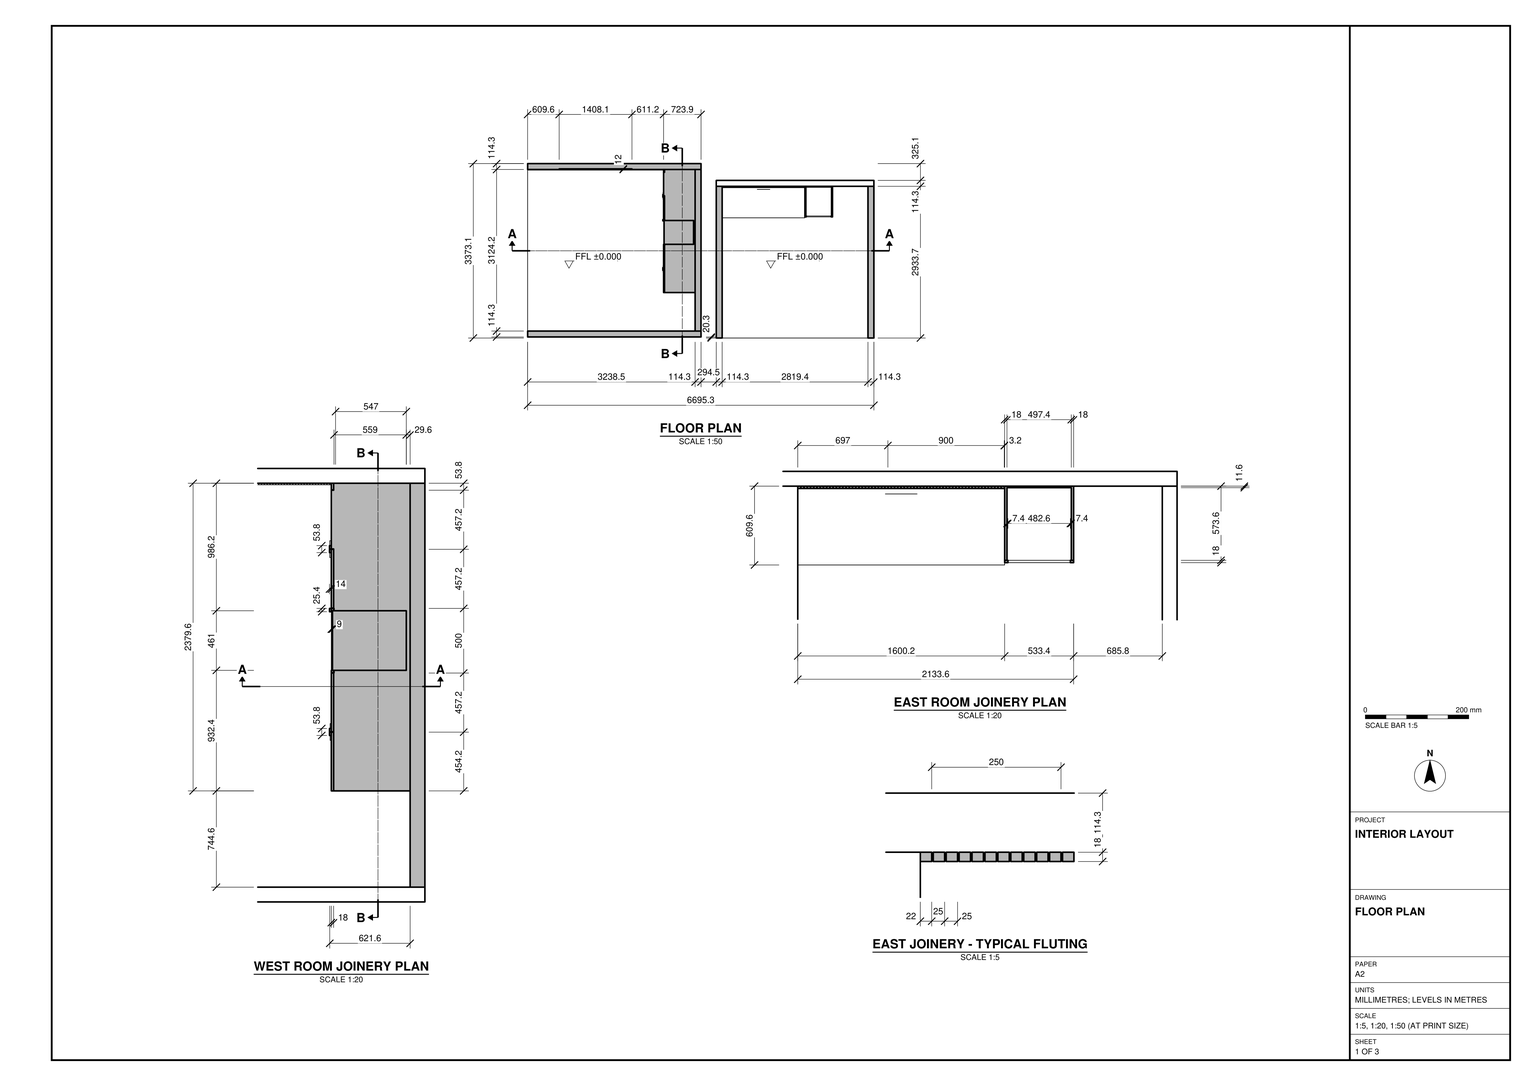
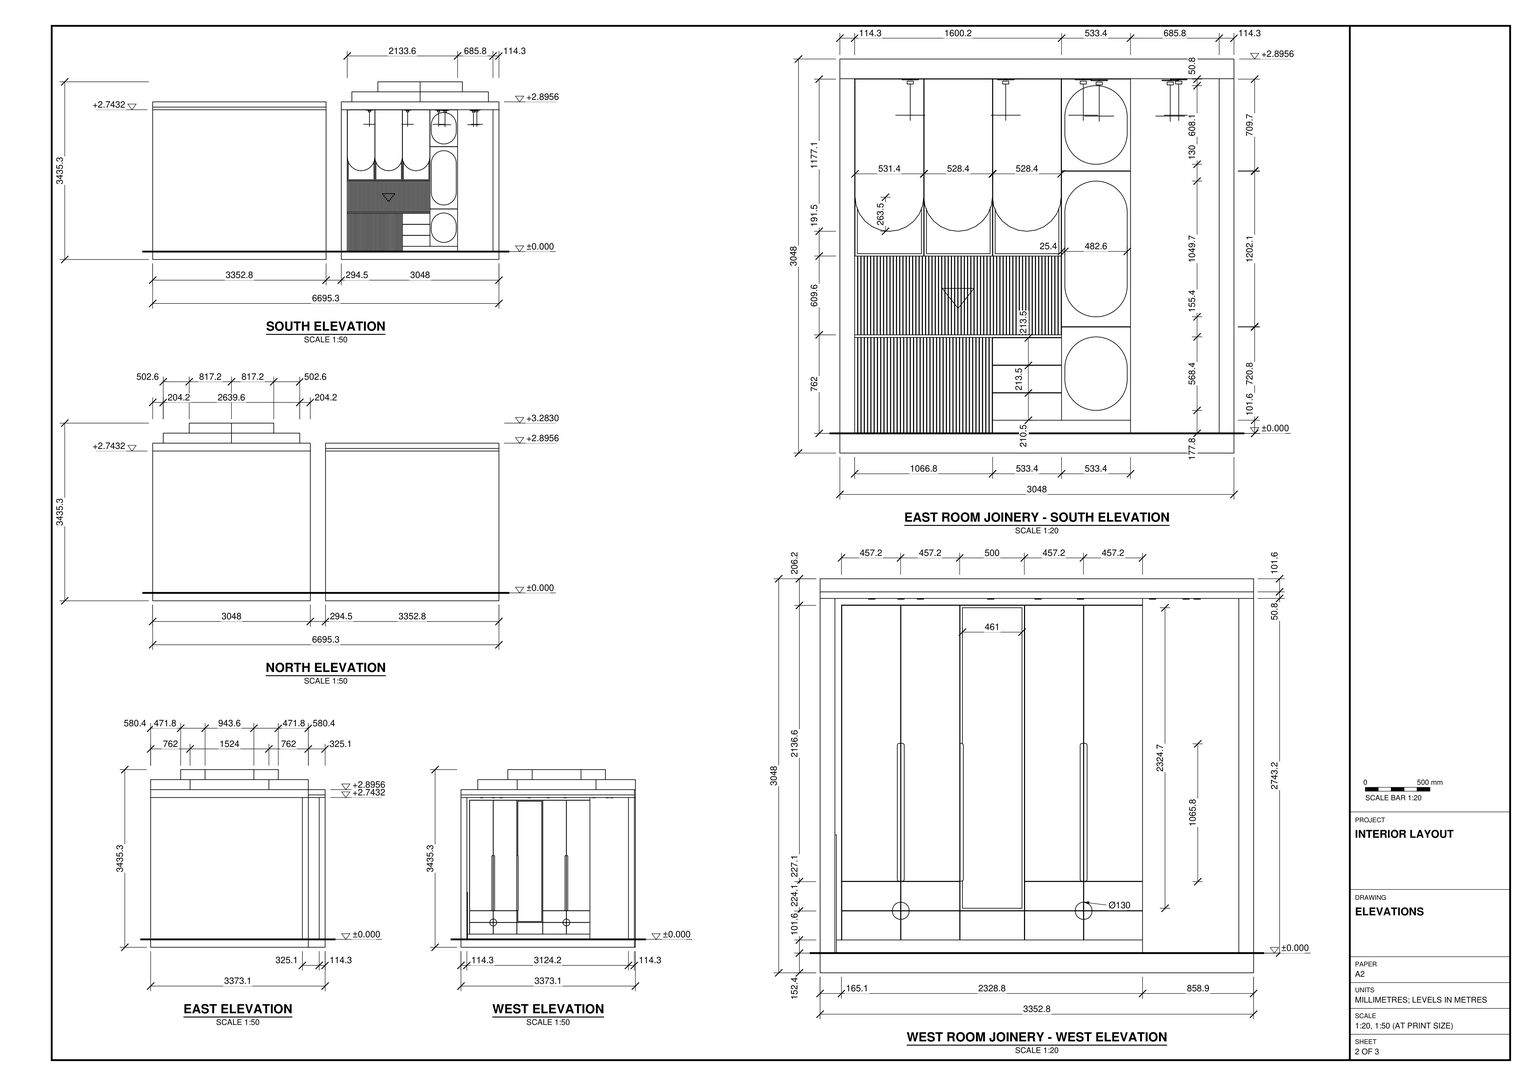
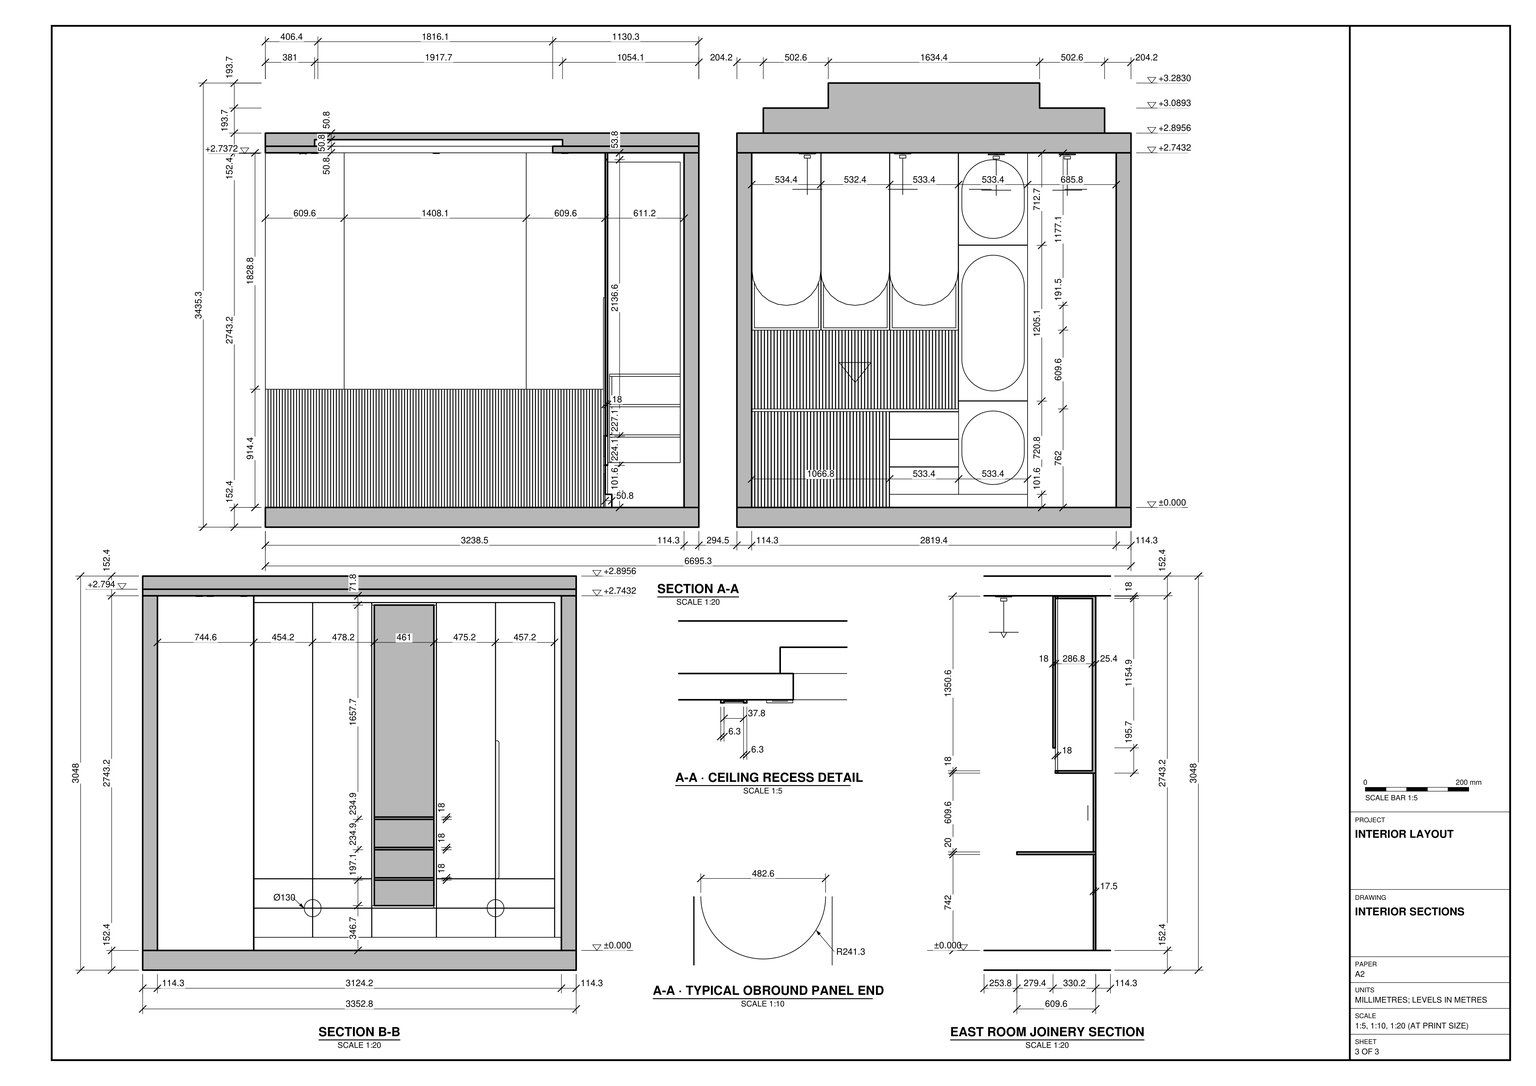
Build the west and east room bays in SketchUp from task_files/diagram_01.pdf. Work in millimetres. The overall model is 6695.3 mm along X, 3373.1 mm along Y and 3435.3 mm high. Both bays have the same finished floor level, ±0.000 (0 mm). Align their south edges, leave the 294.5 mm gap between the shells and set the north edge of the east bay back as drawn. Model the floor slabs, 114.3 mm walls and overhead construction, keeping the west bay open to the west and the east bay open to the south. Follow the sections for the west ceiling recess and the stepped top over the east bay.

Fit the tall storage unit against the east wall of the west bay. Model the paired tall fronts, long pulls, divided lower fronts and framed central bay with its internal shelves. Include the fluted lower wall lining visible in section A-A. Against the north wall of the east bay, build the joinery shown in the south elevation: rounded lower ends on the upper panels, a fluted middle band, a projecting work surface, divided fronts below and a narrow side column with obround panels. Use the enlarged details for the fluting and curved ends. Decor and loose items, including light fixtures, may be any suitable library components placed as shown.

Keep the shell elements and each furniture or joinery piece in separate groups or components, and make repeated parts components. Save one SketchUp model as output_files/two_interior_bays_with_fitted_wall_joinery.skp.

# SketchUp Ruby script. Lengths in millimetres.
U = 1.mm
M = Sketchup.active_model
def pt(a) = Geom::Point3d.new(a.map { |v| v * U })
def face(e, loops, mat)
  f = e.add_face(loops[0].map { |a| pt(a) })
  loops[1..].each { |l| e.add_face(l.map { |a| pt(a) }).erase! }
  f.material = f.back_material = mat if mat
  f
end
# faces: each face lists its corners as indices into pts; further lists are holes
def faces(e, pts, list, mat = nil) = list.each { |f| face(e, (f[0].is_a?(Array) ? f : [f]).map { |l| l.map { |i| pts[i] } }, mat) }
# xy, xz, yz: faces in a plane at the given z, y or x. An outline is a flat list of corners, or four numbers for a rectangle; further outlines are holes
def ring(l) = l.size == 4 ? [[l[0], l[1]], [l[2], l[1]], [l[2], l[3]], [l[0], l[3]]] : l.each_slice(2).to_a
def flat(e, list, mat, &to3) = list.each { |f| face(e, (f[0].is_a?(Array) ? f : [f]).map { |l| ring(l).map { |u, v| to3.(u, v) } }, mat) }
def xy(e, z, list, mat = nil) = flat(e, list, mat) { |x, y| [x, y, z] }
def xz(e, y, list, mat = nil) = flat(e, list, mat) { |x, z| [x, y, z] }
def yz(e, x, list, mat = nil) = flat(e, list, mat) { |y, z| [x, y, z] }
def lines(e, pts, list) = list.each { |a, b| e.add_line(pt(pts[a]), pt(pts[b])) }
# prism: a flat outline (further loops are holes) pulled along v
def prism(e, loops, v, mat = nil)
  f = face(e, loops, mat); d = Geom::Vector3d.new(v.map { |x| x * U })
  f.pushpull(f.normal.samedirection?(d) ? d.length : -d.length)
end
def box(e, o, s, mat = nil) = prism(e, [[o, [o[0] + s[0], o[1], o[2]], [o[0] + s[0], o[1] + s[1], o[2]], [o[0], o[1] + s[1], o[2]]]], [0, 0, s[2]], mat)
def at(x, y, z, deg = 0) = Geom::Transformation.translation(pt([x, y, z])) * Geom::Transformation.rotation(ORIGIN, Z_AXIS, deg.degrees)
def axes(o, x, y, z) = Geom::Transformation.new([*x, 0, *y, 0, *z, 0, *pt(o).to_a, 1])
def part(name) = M.definitions.add(name)
# library, detail: a bought-in or finely detailed component or shape, given as its bounding box
def library(name, o, s) = part(name).tap { |d| box(d.entities, o, s) }
def detail(e, o, s) = box(e.add_group.entities, o, s)
def put(e, d, t, mat = nil) = e.add_instance(d, t).tap { |i| i.material = mat if mat }
def group(e, t, mat = nil) = e.add_group.tap { |g| g.transformation = t; g.material = mat if mat }.entities
root = M.entities
M.materials.add("Olon-Denim-Chic-VT14-1K").color = [84, 100, 105]
M.materials.add("Olon-Fresh-Linen-VT10-1K").color = [226, 220, 209]
M.materials.add("Pionite-a-Panolam-Brand-Canyon-Shadow-SO200-4K").color = [135, 86, 67]
M.materials.add("Uniboard-L17-Ambrette-4K").color = [104, 52, 49]
M.materials.add("Uniboard-L19-Putty-4K").color = [187, 181, 160]
M.materials.add("[Color M00]").color = [255, 255, 255]
M.materials.add("[Color M09]1").color = [0, 0, 0]
M.materials.add("[Translucent Glass Gray]").color = [128, 128, 128]
c1 = part("Group280\#1")
p = [[0,0,0],[0,0,-404.7],[-1.4,0,-404.7],[9,-1301.3,0],[-9,-1301.3,0],[9,1301.3,0],
  [9,0,0],[-9,1301.3,0],[1.4,0,-404.7],[-9,0,0],[0,0,-655.2]]
lines(c1.entities,p,[[0,1],[1,2],[3,4],[5,6],[7,5],[1,8],[9,0],[0,6],[8,10],[4,9],[6,3],[2,10],
  [9,7]])
c2 = part("Rectangle Light\#1")
put(c2.entities,c1,at(0,0,0))
c3 = part("Group282\#1")
p = [[0,0,0],[0,0,-404.7],[-1.4,0,-404.7],[9,-1301.3,0],[-9,-1301.3,0],[9,1301.3,0],
  [9,0,0],[-9,1301.3,0],[1.4,0,-404.7],[-9,0,0],[0,0,-655.2]]
lines(c3.entities,p,[[0,1],[1,2],[3,4],[5,6],[7,5],[1,8],[9,0],[0,6],[8,10],[4,9],[6,3],[2,10],
  [9,7]])
c4 = part("Rectangle Light\#2")
put(c4.entities,c3,at(0,0,0))
c5 = part("Group292\#1")
p = [[0,0,0],[0,0,-167.5],[-81.9,0,-167.5],[533.4,-9,0],[-533.4,-9,0],[533.4,9,0],
  [533.4,0,0],[-533.4,9,0],[81.9,0,-167.5],[-533.4,0,0],[0,0,-271.2]]
lines(c5.entities,p,[[0,1],[1,2],[3,4],[5,6],[7,5],[1,8],[9,0],[0,6],[8,10],[4,9],[6,3],[2,10],
  [9,7]])
c6 = part("Rectangle Light\#3")
put(c6.entities,c5,at(0,0,0))
c7 = library("Group10\#1",[-1313.7,-457.2,0],[2627.4,914.4,12])
c8 = library("Group\#3",[-12,435,0],[621.6,2379.6,2743.2])
c9 = part("Group\#6")
prism(c9.entities,[[[0,248.3,178.4],[0,254.5,178.9],[0,259.6,180.5],[0,263.5,183.1],[0,266.3,186.7],[0,268,191.4],[0,268.6,197.1],[0,461,197.1],[0,461,0],[0,0,0],[0,0,197.1],[0,192.4,197.1],[0,193,191.4],[0,194.7,186.7],[0,197.5,183.1],[0,201.4,180.5],[0,206.5,178.9],[0,212.7,178.4]]],[18,0,0])
c10 = part("Group\#7")
prism(c10.entities,[[[20,25.4,1066.8],[20,17.4,1066.8],[20,12.1,1066.3],[20,7.7,1064.9],[20,4.3,1062.5],[20,1.9,1059.1],[20,0.5,1054.7],[20,0,1049.4],[20,0,17.4],[20,0.5,12.1],[20,1.9,7.7],[20,4.3,4.3],[20,7.7,1.9],[20,12.1,0.5],[20,17.4,0],[20,25.4,0]]],[-14,0,0])
c11 = part("Group\#17")
xy(c11.entities,314.6,[[[110.7,87.8,104.3,89.2,98.4,92.3,93.5,96.8,90,102.4,88,108.7,87.8,115.4,89.2,121.8,92.3,127.7,96.8,132.6,102.4,136.1,108.7,138.1,115.4,138.3,121.8,136.9,127.7,133.8,132.6,129.3,136.1,123.7,138.1,117.3,138.3,110.7,136.9,104.3,133.8,98.4,129.3,93.5,123.7,90,117.3,88],[111.3,94.1,116.3,94.3,121,95.7,125.2,98.4,128.6,102.1,130.9,106.5,132,111.3,131.8,116.3,130.3,121,127.7,125.2,124,128.6,119.6,130.9,114.8,132,109.8,131.8,105.1,130.3,100.9,127.7,97.5,124,95.2,119.6,94.1,114.8,94.3,109.8,95.7,105.1,98.4,100.9,102.1,97.5,106.5,95.2]]])
xy(c11.entities,320.6,[[110.7,87.8,117.3,88,123.7,90,129.3,93.5,133.8,98.4,136.9,104.3,138.3,110.7,138.1,117.3,136.1,123.7,132.6,129.3,127.7,133.8,121.8,136.9,115.4,138.3,108.7,138.1,102.4,136.1,96.8,132.6,92.3,127.7,89.2,121.8,87.8,115.4,88,108.7,90,102.4,93.5,96.8,98.4,92.3,104.3,89.2]])
p = [[110.7,87.8,320.6],[104.3,89.2,320.6],[104.3,89.2,314.6],[110.7,87.8,314.6],[117.3,88,320.6],[117.3,88,314.6],
  [123.7,90,320.6],[123.7,90,314.6],[98.4,92.3,320.6],[98.4,92.3,314.6],[129.3,93.5,320.6],[129.3,93.5,314.6],
  [93.5,96.8,320.6],[93.5,96.8,314.6],[133.8,98.4,320.6],[133.8,98.4,314.6],[111.3,94.1,314.6],[106.5,95.2,314.6],
  [106.5,95.2,317.8],[111.3,94.1,317.8],[116.3,94.3,314.6],[116.3,94.3,317.8],[121,95.7,314.6],[121,95.7,317.8],
  [102.1,97.5,314.6],[102.1,97.5,317.8],[125.2,98.4,314.6],[125.2,98.4,317.8],[90,102.4,320.6],[90,102.4,314.6],
  [98.4,100.9,314.6],[98.4,100.9,317.8],[128.6,102.1,314.6],[128.6,102.1,317.8],[136.9,104.3,320.6],[136.9,104.3,314.6],
  [95.7,105.1,314.6],[95.7,105.1,317.8],[130.9,106.5,314.6],[130.9,106.5,317.8],[88,108.7,320.6],[88,108.7,314.6],
  [138.3,110.7,320.6],[138.3,110.7,314.6],[94.3,109.8,314.6],[94.3,109.8,317.8],[132,111.3,314.6],[132,111.3,317.8],
  [87.8,115.4,320.6],[87.8,115.4,314.6],[94.1,114.8,314.6],[94.1,114.8,317.8],[138.1,117.3,320.6],[138.1,117.3,314.6],
  [131.8,116.3,314.6],[131.8,116.3,317.8],[95.2,119.6,314.6],[95.2,119.6,317.8],[89.2,121.8,320.6],[89.2,121.8,314.6],
  [130.3,121,314.6],[130.3,121,317.8],[136.1,123.7,320.6],[136.1,123.7,314.6],[97.5,124,314.6],[97.5,124,317.8],
  [127.7,125.2,314.6],[127.7,125.2,317.8],[92.3,127.7,320.6],[92.3,127.7,314.6],[132.6,129.3,320.6],[132.6,129.3,314.6],
  [100.9,127.7,314.6],[100.9,127.7,317.8],[124,128.6,314.6],[124,128.6,317.8],[96.8,132.6,320.6],[96.8,132.6,314.6],
  [105.1,130.3,314.6],[105.1,130.3,317.8],[119.6,130.9,314.6],[119.6,130.9,317.8],[127.7,133.8,320.6],[127.7,133.8,314.6],
  [109.8,131.8,314.6],[109.8,131.8,317.8],[114.8,132,314.6],[114.8,132,317.8],[102.4,136.1,320.6],[102.4,136.1,314.6],
  [121.8,136.9,320.6],[121.8,136.9,314.6],[108.7,138.1,320.6],[108.7,138.1,314.6],[115.4,138.3,320.6],[115.4,138.3,314.6]]
faces(c11.entities,p,[[0,1,2,3],[4,0,3,5],[6,4,5,7],[1,8,9,2],[10,6,7,11],[8,12,13,9],[14,10,11,15],[16,17,18,19],
  [20,16,19,21],[22,20,21,23],[17,24,25,18],[26,22,23,27],[12,28,29,13],[24,30,31,25],[32,26,27,33],[34,14,15,35],
  [30,36,37,31],[38,32,33,39],[28,40,41,29],[42,34,35,43],[36,44,45,37],[46,38,39,47],[40,48,49,41],[44,50,51,45],
  [52,42,43,53],[54,46,47,55],[50,56,57,51],[48,58,59,49],[60,54,55,61],[62,52,53,63],[56,64,65,57],[66,60,61,67],
  [58,68,69,59],[70,62,63,71],[64,72,73,65],[74,66,67,75],[68,76,77,69],[72,78,79,73],[80,74,75,81],[82,70,71,83],
  [78,84,85,79],[86,80,81,87],[84,86,87,85],[76,88,89,77],[90,82,83,91],[88,92,93,89],[94,90,91,95],[92,94,95,93]])
g1 = group(c11.entities,at(94.1,94.1,317.8))
xy(g1,0,[[17.2,0,12.4,1.1,8,3.4,4.3,6.8,1.7,11,0.2,15.7,0,20.7,1.1,25.6,3.4,30,6.8,33.6,11,36.3,15.7,37.8,20.7,37.9,25.6,36.8,30,34.5,33.6,31.2,36.3,27,37.8,22.2,37.9,17.2,36.8,12.4,34.5,8,31.2,4.3,27,1.7,22.2,0.2]])
c12 = library("Group161\#1",[-800.1,-304.8,0],[1600.2,609.6,18])
c13 = library("Group227\#2",[-533.4,-371,0],[1066.8,742,17.5])
c14 = part("Group278\#1")
p = [[0,0,0],[0,0,-249.9],[-122.9,0,-249.9],[800.1,-9,0],[-800.1,-9,0],[800.1,9,0],
  [800.1,0,0],[-800.1,9,0],[122.9,0,-249.9],[-800.1,0,0],[0,0,-404.6]]
lines(c14.entities,p,[[0,1],[1,2],[3,4],[5,6],[7,5],[1,8],[9,0],[0,6],[8,10],[4,9],[6,3],[2,10],
  [9,7]])
c15 = part("Rectangle Light")
put(c15.entities,c14,at(0,0,0))
c16 = library("Group\#28",[0,0,0],[533.4,18,709.7])
c17 = library("Group\#29",[0,0,0],[533.4,18,1202.1])
c18 = library("Group\#30",[0,0,0],[533.4,18,720.8])
c19 = library("Group\#31",[0,0,0],[226.1,226.1,320.6])
xy(root,3048,[[5171.3,0,3851.4,762,3851.4,2286,5171.3,3048,6491.1,2286,6491.1,762]])
xy(root,3241.7,[[[5171.3,0,6491.1,762,6491.1,2286,5171.3,3048,3851.4,2286,3851.4,762],[5171.3,580.4,4354.1,1052.2,4354.1,1995.8,5171.3,2467.6,5988.4,1995.8,5988.4,1052.2]]])
xy(root,3435.4,[[5171.3,580.4,5988.4,1052.2,5988.4,1995.8,5171.3,2467.6,4354.1,1995.8,4354.1,1052.2]])
yz(root,2637.9,[[1811.6,499.1,2272.6,2823.8]],"[Translucent Glass Gray]")
yz(root,3851.4,[[762,3048,2286,3241.7]])
yz(root,4354.1,[[1052.2,3241.7,1995.8,3435.4]])
yz(root,5988.4,[[1052.2,3241.7,1995.8,3435.4]])
yz(root,6491.1,[[762,3048,2286,3241.7]])
p = [[3851.4,762,3048],[5171.3,0,3048],[5171.3,0,3241.7],[3851.4,762,3241.7],[6491.1,762,3048],[6491.1,762,3241.7],
  [5171.3,3048,3048],[3851.4,2286,3048],[3851.4,2286,3241.7],[5171.3,3048,3241.7],[6491.1,2286,3048],[6491.1,2286,3241.7],
  [4354.1,1052.2,3241.7],[5171.3,580.4,3241.7],[5171.3,580.4,3435.4],[4354.1,1052.2,3435.4],[5988.4,1052.2,3241.7],[5988.4,1052.2,3435.4],
  [5171.3,2467.6,3241.7],[4354.1,1995.8,3241.7],[4354.1,1995.8,3435.4],[5171.3,2467.6,3435.4],[5988.4,1995.8,3241.7],[5988.4,1995.8,3435.4]]
faces(root,p,[[0,1,2,3],[1,4,5,2],[6,7,8,9],[10,6,9,11],[12,13,14,15],[13,16,17,14],[18,19,20,21],[22,18,21,23]])
put(root,c2,axes([5380,2632.1,1573.3],[0,-1,0],[0,0,1],[-1,0,0]))
put(root,c4,axes([5876.9,2632.1,1573.3],[0,-1,0],[0,0,1],[1,0,0]))
put(root,c6,axes([4295,2858.6,894.1],[1,0,0],[0,-1,0],[0,0,1]))
g2 = group(root,at(0,20.3,0))
box(g2,[0,0,0],[3352.8,3352.8,152.4])
g3 = group(root,at(3238.5,134.6,152.4))
box(g3,[0,0,0],[114.3,3124.2,2743.2])
g4 = group(root,at(0,3258.8,152.4),"Uniboard-L19-Putty-4K")
xy(g4,0,[[0,0,3352.8,114.3]])
xy(g4,2743.2,[[0,0,609.6,0,609.6,12,2017.7,12,2017.7,0,3352.8,0,3352.8,114.3,0,114.3]],"[Color M00]")
xz(g4,0,[[2627.3,0,3352.8,2743.2],[0,914.4,609.6,2743.2],[2017.7,914.4,2627.3,2743.2]])
xz(g4,12,[[609.6,914.4,2017.7,2743.2]])
xz(g4,114.3,[[0,0,3352.8,2743.2]],"[Color M00]")
yz(g4,0,[[0,0,114.3,2743.2]],"[Color M00]")
yz(g4,3352.8,[[0,0,114.3,2743.2]],"[Color M00]")
put(g4,c7,axes([1313.7,0,457.2],[1,0,0],[0,0,1],[0,-1,0]))
g5 = group(g4,at(609.6,0,914.4))
xy(g5,0,[[0,0,1408.1,12]])
yz(g5,0,[[0,0,12,1828.8]],"[Color M00]")
yz(g5,1408.1,[[0,0,12,1828.8]],"[Color M00]")
put(root,c8,at(2628.9,444.2,152.4),"Uniboard-L19-Putty-4K")
g6 = group(root,at(0,20.3,152.4))
box(g6,[0,0,0],[3352.8,114.3,2743.2])
put(root,c9,axes([2661.9,1811.6,952.1],[1,0,0],[0,1,0],[0,0,1.08549]),"Uniboard-L17-Ambrette-4K")
put(root,c9,axes([2661.9,1811.6,717.2],[1,0,0],[0,1,0],[0,0,1.08549]),"Uniboard-L17-Ambrette-4K")
put(root,c9,axes([2661.9,1811.6,505.8],[1,0,0],[0,1,0],[0,0,0.96609]),"Uniboard-L17-Ambrette-4K")
put(root,c10,at(2608.9,1308,708.2),"Uniboard-L17-Ambrette-4K")
put(root,c10,axes([2608.9,1361.8,708.2],[1,0,0],[0,-1,0],[0,0,1]),"Uniboard-L17-Ambrette-4K")
put(root,c10,at(2608.9,2722.4,708.2),"Uniboard-L17-Ambrette-4K")
put(root,c10,axes([2608.9,2776.2,708.2],[1,0,0],[0,-1,0],[0,0,1]),"Uniboard-L17-Ambrette-4K")
put(root,c10,at(2608.9,2265.2,708.2),"[Color M09]1")
g7 = group(root,at(0,20.3,2895.6))
xy(g7,0,[[[0,0,3352.8,3352.8],[631.1,520.7,1997.8,520.7,2066.4,526.9,2122.6,545.7,2166.3,576.9,2197.5,620.6,2216.3,676.8,2222.5,745.4,2222.5,2619.4,2216.3,2688,2197.5,2744.2,2166.3,2787.9,2122.6,2819.1,2066.4,2837.9,1997.8,2844.1,631.1,2844.1,562.5,2837.9,506.3,2819.1,462.6,2787.9,431.4,2744.2,412.6,2688,406.4,2619.4,406.4,745.4,412.6,676.8,431.4,620.6,462.6,576.9,506.3,545.7,562.5,526.9]]])
xy(g7,50.8,[[[0,0,3352.8,3352.8],[381,495.3,2298.7,2869.5]],[381,495.3,2222.5,520.7],[2222.5,495.3,2298.7,2844.1],[381,520.7,406.4,2844.1],[406.4,520.7,631.1,520.7,562.5,526.9,506.3,545.7,462.6,576.9,431.4,620.6,412.6,676.8,406.4,745.4],
  [1997.8,520.7,2222.5,520.7,2222.5,745.4,2216.3,676.8,2197.5,620.6,2166.3,576.9,2122.6,545.7,2066.4,526.9],[406.4,2619.4,412.6,2688,431.4,2744.2,462.6,2787.9,506.3,2819.1,562.5,2837.9,631.1,2844.1,406.4,2844.1],[2222.5,2619.4,2222.5,2844.1,1997.8,2844.1,2066.4,2837.9,2122.6,2819.1,2166.3,2787.9,2197.5,2744.2,2216.3,2688],[381,2844.1,2298.7,2869.5]])
xy(g7,101.6,[[381,495.3,2298.7,2869.5]])
xy(g7,152.4,[[0,0,3352.8,3352.8]])
xz(g7,0,[[0,0,3352.8,50.8],[0,50.8,3352.8,152.4]])
xz(g7,520.7,[[631.1,0,1997.8,50.8]])
xz(g7,2844.1,[[631.1,0,1997.8,50.8]])
xz(g7,3352.8,[[0,0,3352.8,50.8],[0,50.8,3352.8,152.4]])
yz(g7,0,[[0,0,3352.8,50.8],[0,50.8,3352.8,152.4]])
yz(g7,406.4,[[745.4,0,2619.4,50.8]])
yz(g7,2222.5,[[745.4,0,2619.4,50.8]])
yz(g7,3352.8,[[0,0,3352.8,50.8],[0,50.8,3352.8,152.4]])
p = [[631.1,520.7,50.8],[631.1,520.7,0],[562.5,526.9,0],[562.5,526.9,50.8],[1997.8,520.7,0],[1997.8,520.7,50.8],
  [2066.4,526.9,50.8],[2066.4,526.9,0],[506.3,545.7,0],[506.3,545.7,50.8],[2122.6,545.7,50.8],[2122.6,545.7,0],
  [462.6,576.9,0],[462.6,576.9,50.8],[2166.3,576.9,50.8],[2166.3,576.9,0],[431.4,620.6,0],[431.4,620.6,50.8],
  [2197.5,620.6,50.8],[2197.5,620.6,0],[412.6,676.8,0],[412.6,676.8,50.8],[2216.3,676.8,50.8],[2216.3,676.8,0],
  [406.4,745.4,0],[406.4,745.4,50.8],[2222.5,745.4,50.8],[2222.5,745.4,0],[406.4,2619.4,50.8],[406.4,2619.4,0],
  [412.6,2688,0],[412.6,2688,50.8],[2216.3,2688,50.8],[2216.3,2688,0],[2222.5,2619.4,0],[2222.5,2619.4,50.8],
  [431.4,2744.2,0],[431.4,2744.2,50.8],[2197.5,2744.2,50.8],[2197.5,2744.2,0],[462.6,2787.9,0],[462.6,2787.9,50.8],
  [2166.3,2787.9,50.8],[2166.3,2787.9,0],[506.3,2819.1,0],[506.3,2819.1,50.8],[2122.6,2819.1,50.8],[2122.6,2819.1,0],
  [562.5,2837.9,0],[562.5,2837.9,50.8],[2066.4,2837.9,50.8],[2066.4,2837.9,0],[631.1,2844.1,0],[631.1,2844.1,50.8],
  [1997.8,2844.1,50.8],[1997.8,2844.1,0]]
faces(g7,p,[[0,1,2,3],[4,5,6,7],[3,2,8,9],[7,6,10,11],[9,8,12,13],[11,10,14,15],[13,12,16,17],[15,14,18,19],
  [17,16,20,21],[19,18,22,23],[21,20,24,25],[23,22,26,27],[28,29,30,31],[32,33,34,35],[31,30,36,37],[38,39,33,32],
  [37,36,40,41],[42,43,39,38],[41,40,44,45],[46,47,43,42],[45,44,48,49],[50,51,47,46],[49,48,52,53],[54,55,51,50]])
g8 = group(g7,at(2298.7,495.3,50.8))
yz(g8,0,[[0,0,2374.2,50.8]])
g9 = group(g7,at(381,2869.5,50.8))
xz(g9,0,[[0,0,1917.7,50.8]])
g10 = group(g7,at(381,495.3,50.8))
xz(g10,0,[[0,0,1917.7,50.8]])
g11 = group(g7,at(381,495.3,50.8))
yz(g11,0,[[0,0,2374.2,50.8]])
put(root,c11,at(2203.5,2634.6,2575))
put(root,c11,at(2203.5,1245.5,2575))
put(root,c11,at(2203.5,1940.8,2575))
put(root,c11,at(2725.8,429.5,2575))
put(root,c11,at(1824.2,343.8,2575))
put(root,c11,at(570,343.8,2575))
put(root,c11,at(1197.1,343.8,2575))
put(root,c11,at(1208.6,2860.3,2575))
put(root,c11,at(267.2,2860.3,2575))
put(root,c11,at(178.3,1574.5,2575))
put(root,c11,at(178.3,688.6,2575))
put(root,c11,at(178.3,2484.1,2575))
g12 = group(root,at(3647.3,0,0))
box(g12,[0,0,0],[3048,3048,152.4])
g13 = group(g12,at(2933.7,0,152.4))
box(g13,[0,0,0],[114.3,2933.7,2743.2])
g14 = group(g12,at(0,0,152.4))
box(g14,[0,0,0],[114.3,2933.7,2743.2])
g15 = group(root,at(3647.3,2933.7,152.4))
xy(g15,0,[[0,0,3048,114.3]])
xy(g15,2743.2,[[0,0,3048,114.3]])
xz(g15,0,[[[0,0,114.3,0,114.3,742,1181.1,742,1181.1,0,3048,0,3048,2743.2,0,2743.2],[114.3,762,1714.5,1371.6]]])
xz(g15,114.3,[[0,0,3048,2743.2]])
yz(g15,0,[[0,0,114.3,2743.2]])
yz(g15,3048,[[0,0,114.3,2743.2]])
put(g15,c12,axes([914.4,0,1066.8],[1,0,0],[0,0,1],[0,-1,0]),"Olon-Denim-Chic-VT14-1K")
put(g15,c13,axes([647.7,0,371],[1,0,0],[0,0,1],[0,-1,0]),"Olon-Denim-Chic-VT14-1K")
g16 = group(root,at(3761.6,2324.1,152.4),"Olon-Fresh-Linen-VT10-1K")
xy(g16,0,[[1066.8,50.8,2133.6,609.6]])
xy(g16,101.6,[[1066.8,0,1600.2,18],[1066.8,18,1600.2,50.8],[1600.2,36,2133.6,50.8]])
xy(g16,119.6,[[1618.2,36,2115.6,598]],"Pionite-a-Panolam-Brand-Canyon-Shadow-SO200-4K")
xy(g16,312.1,[[1066.8,0,1600.2,18]])
xy(g16,315.1,[[1066.8,0,1600.2,18]])
xy(g16,525.5,[[1066.8,0,1600.2,18]])
xy(g16,528.5,[[1066.8,0,1600.2,18]])
xy(g16,739,[[1066.8,0,1600.2,18]])
xy(g16,742,[[0,0,1066.8,609.6],[1066.8,0,1600.2,18]])
xy(g16,762,[[0,0,1600.2,609.6]])
xy(g16,805.9,[[1618.2,36,2115.6,598]],"Pionite-a-Panolam-Brand-Canyon-Shadow-SO200-4K")
xy(g16,841.9,[[1618.2,36,2115.6,598]],"Pionite-a-Panolam-Brand-Canyon-Shadow-SO200-4K")
xy(g16,2011,[[1618.2,36,2115.6,598]],"Pionite-a-Panolam-Brand-Canyon-Shadow-SO200-4K")
xy(g16,2047,[[1618.2,36,2115.6,598]],"Pionite-a-Panolam-Brand-Canyon-Shadow-SO200-4K")
xy(g16,2722.2,[[1618.2,36,2115.6,598]],"Pionite-a-Panolam-Brand-Canyon-Shadow-SO200-4K")
xy(g16,2740.2,[[1600.2,36,2133.6,609.6]])
xz(g16,0,[[1066.8,101.6,1600.2,312.1],[1066.8,315.1,1600.2,525.5],[1066.8,528.5,1600.2,739],[0,742,1600.2,762]])
xz(g16,18,[[1066.8,101.6,1600.2,312.1],[1066.8,312.1,1600.2,315.1],[1066.8,315.1,1600.2,525.5],[1066.8,525.5,1600.2,528.5],[1066.8,528.5,1600.2,739],
  [1066.8,739,1600.2,742]])
xz(g16,36,[[[1600.2,101.6,2133.6,823.9],[1618.2,119.6,2115.6,805.9]],[[1600.2,823.9,2133.6,2029],[1618.2,841.9,2115.6,2011]],[[1600.2,2029,2133.6,2740.2],[1618.2,2047,2115.6,2722.2]]])
xz(g16,50.8,[[1066.8,0,2133.6,101.6]])
xz(g16,598,[[1618.2,119.6,2115.6,805.9],[1618.2,841.9,2115.6,2011],[1618.2,2047,2115.6,2722.2]],"Pionite-a-Panolam-Brand-Canyon-Shadow-SO200-4K")
xz(g16,609.6,[[1066.8,0,1066.8,742,0,742,0,762,1600.2,762,1600.2,2740.2,2133.6,2740.2,2133.6,0]])
yz(g16,0,[[0,742,609.6,762]])
yz(g16,1066.8,[[50.8,0,50.8,101.6,18,101.6,18,742,609.6,742,609.6,0],[0,101.6,18,312.1],[0,315.1,18,525.5],[0,528.5,18,739]])
yz(g16,1600.2,[[0,101.6,18,312.1],[18,101.6,36,312.1],[18,312.1,36,315.1],[0,315.1,18,525.5],[18,315.1,36,525.5],
  [18,525.5,36,528.5],[0,528.5,18,739],[18,528.5,36,739],[18,739,36,742],[0,742,36,762],
  [36,762,609.6,2740.2]])
yz(g16,1618.2,[[36,119.6,598,739],[36,739,598,742],[36,742,598,762],[36,762,598,805.9],[36,841.9,598,2011],
  [36,2047,598,2722.2]],"Pionite-a-Panolam-Brand-Canyon-Shadow-SO200-4K")
yz(g16,2115.6,[[36,119.6,598,805.9],[36,841.9,598,2011],[36,2047,598,2722.2]],"Pionite-a-Panolam-Brand-Canyon-Shadow-SO200-4K")
yz(g16,2133.6,[[50.8,0,609.6,0,609.6,2740.2,36,2740.2,36,101.6,50.8,101.6]])
g17 = group(root,at(3761.6,2578.1,1524),"Olon-Fresh-Linen-VT10-1K")
xy(g17,0,[[1068.8,43.4,1597.2,61.4]],"Olon-Denim-Chic-VT14-1K")
xy(g17,0,[[3,43.4,534.4,61.4],[537.4,43.4,1065.8,61.4],[0,56.1,0,355.6,1600.2,355.6,1600.2,56.1,1597.2,56.1,1597.2,61.4,1068.8,61.4,1068.8,60.9,1065.8,60.9,1065.8,61.4,537.4,61.4,537.4,78.9,534.4,78.9,534.4,61.4,3,61.4,3,56.1]],"Pionite-a-Panolam-Brand-Canyon-Shadow-SO200-4K")
xy(g17,18,[[21,43.4,516.4,61.4],[555.4,43.4,1047.8,61.4],[1086.8,43.4,1579.2,61.4],[21,61.4,516.4,330.2],[555.4,61.4,1047.8,330.2],
  [1086.8,61.4,1579.2,330.2]],"Pionite-a-Panolam-Brand-Canyon-Shadow-SO200-4K")
xy(g17,1350.6,[[21,61.4,516.4,330.2],[555.4,61.4,1047.8,330.2],[1086.8,61.4,1579.2,330.2]])
xy(g17,1350.6,[[21,43.4,516.4,61.4],[555.4,43.4,1047.8,61.4],[1086.8,43.4,1579.2,61.4]],"Olon-Denim-Chic-VT14-1K")
xy(g17,1368.6,[[0,56.1,3,56.1,3,61.4,534.4,61.4,534.4,78.9,537.4,78.9,537.4,61.4,1065.8,61.4,1065.8,60.9,1068.8,60.9,1068.8,61.4,1597.2,61.4,1597.2,56.1,1600.2,56.1,1600.2,355.6,0,355.6]])
xy(g17,1368.6,[[3,43.4,534.4,61.4],[537.4,43.4,1065.8,61.4],[1068.8,43.4,1597.2,61.4]],"Olon-Denim-Chic-VT14-1K")
xz(g17,43.4,[[[3,0,534.4,1368.6],[21,18,516.4,1350.6]],[[537.4,0,1065.8,1368.6],[555.4,18,1047.8,1350.6]],[[1068.8,0,1597.2,1368.6],[1086.8,18,1579.2,1350.6]]],"Pionite-a-Panolam-Brand-Canyon-Shadow-SO200-4K")
xz(g17,56.1,[[0,0,3,1368.6],[1597.2,0,1600.2,1368.6]])
xz(g17,60.9,[[1065.8,0,1068.8,1368.6]])
xz(g17,61.4,[[[3,0,534.4,1368.6],[21,18,516.4,1350.6]],[[537.4,0,1065.8,1368.6],[555.4,18,1047.8,1350.6]],[[1068.8,0,1597.2,1368.6],[1086.8,18,1579.2,1350.6]]],"Olon-Denim-Chic-VT14-1K")
xz(g17,78.9,[[534.4,0,537.4,1368.6]])
xz(g17,330.2,[[21,18,516.4,1350.6],[555.4,18,1047.8,1350.6],[1086.8,18,1579.2,1350.6]],"Pionite-a-Panolam-Brand-Canyon-Shadow-SO200-4K")
xz(g17,355.6,[[0,0,1600.2,1368.6]])
yz(g17,0,[[56.1,0,355.6,1368.6]])
yz(g17,3,[[56.1,0,61.4,1368.6]],"Olon-Denim-Chic-VT14-1K")
yz(g17,3,[[43.4,0,56.1,1368.6]],"Pionite-a-Panolam-Brand-Canyon-Shadow-SO200-4K")
yz(g17,21,[[43.4,18,61.4,1350.6],[61.4,18,330.2,1350.6]],"Pionite-a-Panolam-Brand-Canyon-Shadow-SO200-4K")
yz(g17,516.4,[[43.4,18,61.4,1350.6],[61.4,18,330.2,1350.6]],"Pionite-a-Panolam-Brand-Canyon-Shadow-SO200-4K")
yz(g17,534.4,[[61.4,0,78.9,1368.6]],"Olon-Denim-Chic-VT14-1K")
yz(g17,534.4,[[43.4,0,61.4,1368.6]],"Pionite-a-Panolam-Brand-Canyon-Shadow-SO200-4K")
yz(g17,537.4,[[61.4,0,78.9,1368.6]],"Olon-Denim-Chic-VT14-1K")
yz(g17,537.4,[[43.4,0,61.4,1368.6]],"Pionite-a-Panolam-Brand-Canyon-Shadow-SO200-4K")
yz(g17,555.4,[[43.4,18,61.4,1350.6],[61.4,18,330.2,1350.6]],"Pionite-a-Panolam-Brand-Canyon-Shadow-SO200-4K")
yz(g17,1047.8,[[43.4,18,61.4,1350.6],[61.4,18,330.2,1350.6]],"Pionite-a-Panolam-Brand-Canyon-Shadow-SO200-4K")
yz(g17,1065.8,[[43.4,0,60.9,1368.6],[60.9,0,61.4,1368.6]],"Olon-Denim-Chic-VT14-1K")
yz(g17,1068.8,[[60.9,0,61.4,1368.6]],"Olon-Denim-Chic-VT14-1K")
yz(g17,1068.8,[[43.4,0,60.9,1368.6]],"Pionite-a-Panolam-Brand-Canyon-Shadow-SO200-4K")
yz(g17,1086.8,[[43.4,18,61.4,1350.6],[61.4,18,330.2,1350.6]],"Pionite-a-Panolam-Brand-Canyon-Shadow-SO200-4K")
yz(g17,1579.2,[[43.4,18,61.4,1350.6],[61.4,18,330.2,1350.6]],"Pionite-a-Panolam-Brand-Canyon-Shadow-SO200-4K")
yz(g17,1597.2,[[43.4,0,56.1,1368.6],[56.1,0,61.4,1368.6]],"Olon-Denim-Chic-VT14-1K")
yz(g17,1600.2,[[56.1,0,355.6,1368.6]])
put(g17,c15,at(800.1,295.3,-0.3,180))
g18 = group(g17,at(3,25.4,0))
prism(g18,[[[0,18,1368.6],[531.4,18,1368.6],[531.4,18,457.2],[522.3,18,388.4],[495.8,18,324.3],[453.6,18,269.3],[398.6,18,227.1],[334.5,18,200.6],[265.7,18,191.5],[196.9,18,200.6],[132.9,18,227.1],[77.8,18,269.3],[35.6,18,324.3],[9.1,18,388.4],[0,18,457.2]]],[0,-18,0])
g19 = group(g17,at(534.4,0,191.5))
prism(g19,[[[3,43.4,242.9],[3,43.4,1177.1],[531.4,43.4,1177.1],[531.4,43.4,265.7],[522.3,43.4,196.9],[495.8,43.4,132.9],[453.6,43.4,77.8],[398.5,43.4,35.6],[334.5,43.4,9.1],[265.7,43.4,0],[196.9,43.4,9.1],[132.9,43.4,35.6],[77.8,43.4,77.8],[35.6,43.4,132.8],[9.1,43.4,196.9]]],[0,-18,0])
# 1 loose lines left out
g20 = group(g17,at(1065.8,0,191.5))
prism(g20,[[[3,43.4,242.9],[3,43.4,1177.1],[531.4,43.4,1177.1],[531.4,43.4,265.7],[522.3,43.4,196.9],[495.8,43.4,132.9],[453.6,43.4,77.8],[398.5,43.4,35.6],[334.5,43.4,9.1],[265.7,43.4,0],[196.9,43.4,9.1],[132.9,43.4,35.6],[77.8,43.4,77.8],[35.6,43.4,132.8],[9.1,43.4,196.9]]],[0,-18,0])
# 1 loose lines left out
put(root,c16,at(5361.8,2342.1,2182.9),"Olon-Fresh-Linen-VT10-1K")
put(root,c17,at(5361.8,2342.1,977.8),"Olon-Fresh-Linen-VT10-1K")
put(root,c18,at(5361.8,2342.1,254),"Olon-Fresh-Linen-VT10-1K")
g21 = group(root,at(3647.3,0,2895.6))
box(g21,[0,0,0],[3048,3048,152.4])
put(root,c19,at(4078.6,2109.5,2572))
put(root,c19,at(4816.8,2109.5,2572))
put(root,c19,at(6089.4,2462.9,2565.1))
put(root,c19,at(5540,1875.3,2565.1))
put(root,c19,at(4078.6,1499.9,2572))
put(root,c19,at(4816.8,1499.9,2572))
put(root,c19,at(4078.6,890.3,2572))
put(root,c19,at(4816.8,890.3,2572))
put(root,c19,at(4078.6,280.7,2572))
put(root,c19,at(4816.8,280.7,2572))
put(root,c19,at(5416.9,1499.9,2572))
put(root,c19,at(6155.1,1499.9,2572))
put(root,c19,at(5416.9,280.7,2572))
put(root,c19,at(5416.9,890.3,2572))
put(root,c19,at(6155.1,280.7,2572))
put(root,c19,at(6155.1,890.3,2572))
